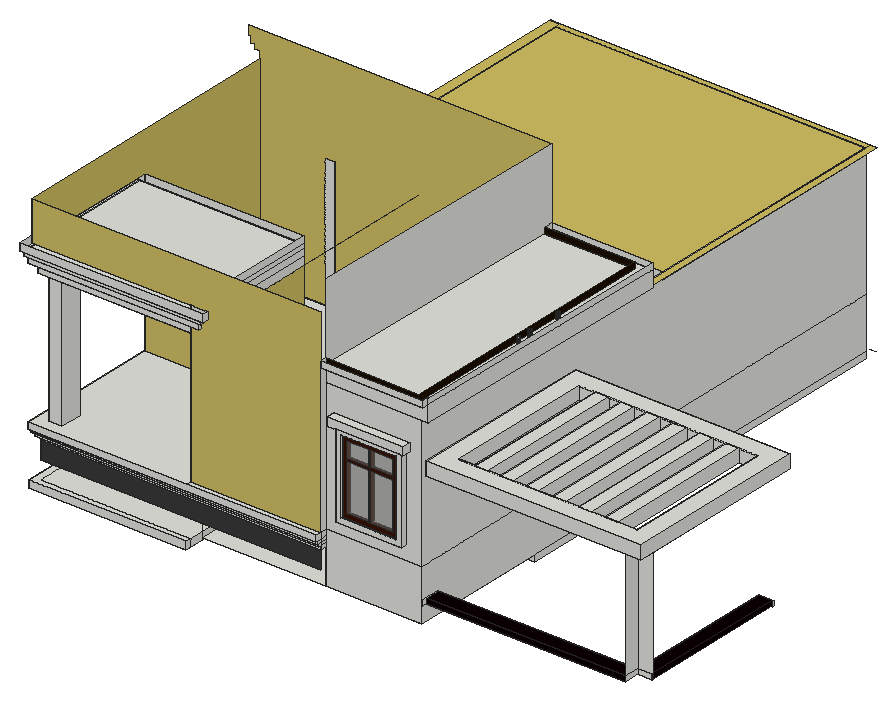
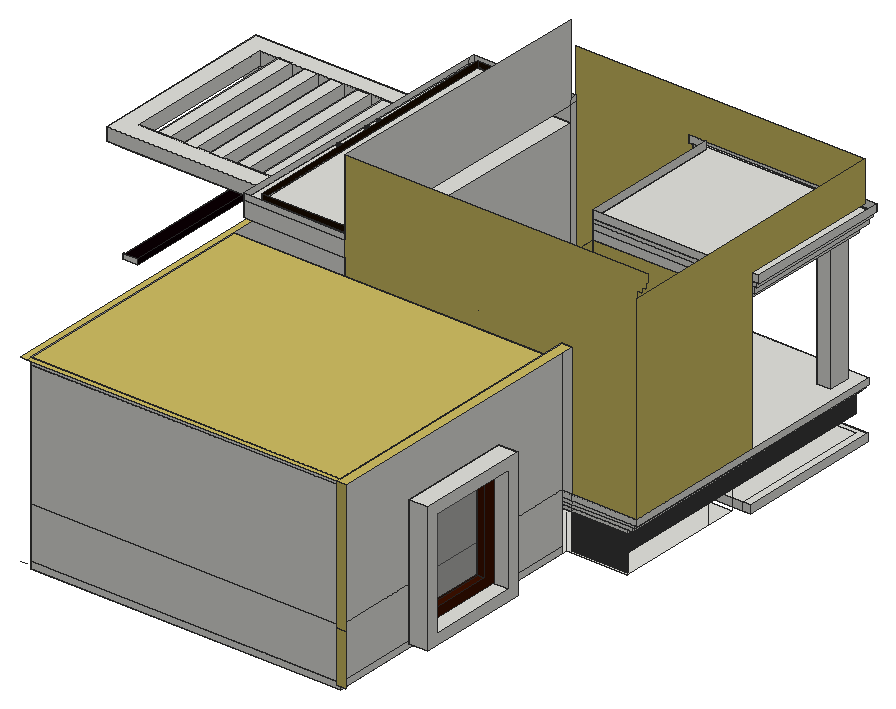
# SketchUp Ruby script. Lengths in inches.
U = 1.inch
M = Sketchup.active_model
def pt(a) = Geom::Point3d.new(a.map { |v| v * U })
def face(e, loops, mat)
  f = e.add_face(loops[0].map { |a| pt(a) })
  loops[1..].each { |l| e.add_face(l.map { |a| pt(a) }).erase! }
  f.material = f.back_material = mat if mat
  f
end
# faces: each face lists its corners as indices into pts; further lists are holes
def faces(e, pts, list, mat = nil) = list.each { |f| face(e, (f[0].is_a?(Array) ? f : [f]).map { |l| l.map { |i| pts[i] } }, mat) }
# xy, xz, yz: faces in a plane at the given z, y or x. An outline is a flat list of corners, or four numbers for a rectangle; further outlines are holes
def ring(l) = l.size == 4 ? [[l[0], l[1]], [l[2], l[1]], [l[2], l[3]], [l[0], l[3]]] : l.each_slice(2).to_a
def flat(e, list, mat, &to3) = list.each { |f| face(e, (f[0].is_a?(Array) ? f : [f]).map { |l| ring(l).map { |u, v| to3.(u, v) } }, mat) }
def xy(e, z, list, mat = nil) = flat(e, list, mat) { |x, y| [x, y, z] }
def xz(e, y, list, mat = nil) = flat(e, list, mat) { |x, z| [x, y, z] }
def yz(e, x, list, mat = nil) = flat(e, list, mat) { |y, z| [x, y, z] }
def lines(e, pts, list) = list.each { |a, b| e.add_line(pt(pts[a]), pt(pts[b])) }
# prism: a flat outline (further loops are holes) pulled along v
def prism(e, loops, v, mat = nil)
  f = face(e, loops, mat); d = Geom::Vector3d.new(v.map { |x| x * U })
  f.pushpull(f.normal.samedirection?(d) ? d.length : -d.length)
end
def box(e, o, s, mat = nil) = prism(e, [[o, [o[0] + s[0], o[1], o[2]], [o[0] + s[0], o[1] + s[1], o[2]], [o[0], o[1] + s[1], o[2]]]], [0, 0, s[2]], mat)
def at(x, y, z, deg = 0) = Geom::Transformation.translation(pt([x, y, z])) * Geom::Transformation.rotation(ORIGIN, Z_AXIS, deg.degrees)
def axes(o, x, y, z) = Geom::Transformation.new([*x, 0, *y, 0, *z, 0, *pt(o).to_a, 1])
def part(name) = M.definitions.add(name)
# library, detail: a bought-in or finely detailed component or shape, given as its bounding box
def library(name, o, s) = part(name).tap { |d| box(d.entities, o, s) }
def detail(e, o, s) = box(e.add_group.entities, o, s)
def put(e, d, t, mat = nil) = e.add_instance(d, t).tap { |i| i.material = mat if mat }
def group(e, t, mat = nil) = e.add_group.tap { |g| g.transformation = t; g.material = mat if mat }.entities
root = M.entities
M.materials.add("[Color C08]").color = [60, 17, 0]
M.materials.add("[Color D05]").color = [208, 191, 99]
M.materials.add("[Color E01]").color = [255, 255, 204]
M.materials.add("[Color M07]").color = [58, 58, 58]
M.materials.add("[Metal Seamed]").color = [11, 0, 4]
M.materials.add("[Metal Seamed]1").color = [28, 14, 0]
M.materials.add("[Translucent Glass Gray]").color = [128, 128, 128]
M.materials["[Translucent Glass Gray]"].alpha = 0.5
M.materials.add("[Wood Cherry Original]").color = [152, 86, 42]
c1 = part("Group\#2")
xy(c1.entities,0,[[0,0,43.625,4]],"[Color C08]")
xy(c1.entities,4.9,[[4.9,0,38.73,4]],"[Color C08]")
xy(c1.entities,53.48,[[4.9,0,38.73,4]],"[Color C08]")
xy(c1.entities,58.375,[[0,0,43.625,4]],"[Color C08]")
xz(c1.entities,0,[[[0,0,43.625,58.375],[4.9,4.9,38.73,53.48]]],"[Color C08]")
xz(c1.entities,0,[[4.9,4.9,38.73,53.48]],"[Translucent Glass Gray]")
xz(c1.entities,4,[[[0,0,43.625,58.375],[4.9,4.9,38.73,53.48]]],"[Color C08]")
yz(c1.entities,0,[[0,0,4,58.375]],"[Color C08]")
yz(c1.entities,4.9,[[0,4.9,4,53.48]],"[Color C08]")
yz(c1.entities,38.73,[[0,4.9,4,53.48]],"[Color C08]")
yz(c1.entities,43.625,[[0,0,4,58.375]],"[Color C08]")
c2 = part("Group\#1")
xy(c2.entities,0,[[0,0,6.3125,48]],"[Wood Cherry Original]")
xy(c2.entities,4.83,[[2.3125,4.83,3.9375,43.17]])
xy(c2.entities,4.83,[[0,4.83,2.3125,43.17],[3.9375,4.83,6.3125,43.17]],"[Wood Cherry Original]")
xy(c2.entities,79.17,[[2.3125,4.83,3.9375,43.17]])
xy(c2.entities,79.17,[[0,4.83,2.3125,43.17],[3.9375,4.83,6.3125,43.17]],"[Wood Cherry Original]")
xy(c2.entities,84,[[0,0,6.3125,48]],"[Wood Cherry Original]")
xz(c2.entities,0,[[0,0,6.3125,84]],"[Wood Cherry Original]")
xz(c2.entities,4.83,[[2.3125,4.83,3.9375,79.17]])
xz(c2.entities,4.83,[[0,4.83,2.3125,79.17],[3.9375,4.83,6.3125,79.17]],"[Wood Cherry Original]")
xz(c2.entities,43.17,[[2.3125,4.83,3.9375,79.17]])
xz(c2.entities,43.17,[[0,4.83,2.3125,79.17],[3.9375,4.83,6.3125,79.17]],"[Wood Cherry Original]")
xz(c2.entities,48,[[0,0,6.3125,84]],"[Wood Cherry Original]")
yz(c2.entities,0,[[[0,0,48,84],[4.83,4.83,43.17,79.17]]],"[Wood Cherry Original]")
yz(c2.entities,2.3125,[[7.68,9.76,40.37,11.76],[7.68,18.32,40.37,20.32],[7.68,27.01,40.37,29.01],[7.68,35.69,40.37,37.69],[7.68,44.38,40.37,46.38],
  [7.68,53.07,40.37,55.07],[7.68,61.76,40.37,63.76],[7.68,70.44,40.37,72.44]],"[Color E01]")
yz(c2.entities,2.3125,[[[4.83,4.83,43.17,79.17],[7.68,70.44,40.37,72.44],[7.68,61.76,40.37,63.76],[7.68,53.07,40.37,55.07],[7.68,44.38,40.37,46.38],[7.68,35.69,40.37,37.69],[7.68,27.01,40.37,29.01],[7.68,18.32,40.37,20.32],[7.68,9.76,40.37,11.76]]],"[Wood Cherry Original]")
yz(c2.entities,3.9375,[[4.83,4.83,43.17,79.17]],"[Wood Cherry Original]")
yz(c2.entities,6.3125,[[[0,0,48,84],[4.83,4.83,43.17,79.17]]],"[Wood Cherry Original]")
c3 = part("Group\#3")
xy(c3.entities,0,[[0,0,51.6875,4]],"[Color C08]")
xy(c3.entities,4.05,[[4.05,0,24.41,4],[24.41,0,26.55,4],[26.55,0,47.64,4]],"[Color C08]")
xy(c3.entities,49.59,[[4.05,0,24.41,4],[26.55,0,47.64,4]],"[Color C08]")
xy(c3.entities,51.6875,[[4.05,0,24.41,4],[26.55,0,47.64,4]],"[Color C08]")
xy(c3.entities,67.57,[[4.05,0,24.41,4],[26.55,0,47.64,4]],"[Color C08]")
xy(c3.entities,71.625,[[0,0,51.6875,4]],"[Color C08]")
xz(c3.entities,0,[[[0,0,51.6875,71.625],[4.05,4.05,4.05,49.59,24.41,49.59,24.41,4.05,26.55,4.05,26.55,49.59,47.64,49.59,47.64,4.05],[26.55,51.6875,47.64,67.57],[4.05,51.6875,24.41,67.57]]],"[Color C08]")
xz(c3.entities,0,[[4.05,4.05,24.41,49.59],[26.55,4.05,47.64,49.59],[4.05,51.6875,24.41,67.57],[26.55,51.6875,47.64,67.57]],"[Translucent Glass Gray]")
xz(c3.entities,4,[[[0,0,51.6875,71.625],[4.05,4.05,4.05,49.59,24.41,49.59,24.41,4.05,26.55,4.05,26.55,49.59,47.64,49.59,47.64,4.05],[26.55,51.6875,47.64,67.57],[4.05,51.6875,24.41,67.57]]],"[Color C08]")
yz(c3.entities,0,[[0,0,4,71.625]],"[Color C08]")
yz(c3.entities,4.05,[[0,4.05,4,49.59],[0,51.6875,4,67.57]],"[Color C08]")
yz(c3.entities,24.41,[[0,4.05,4,49.59],[0,51.6875,4,67.57]],"[Color C08]")
yz(c3.entities,26.55,[[0,4.05,4,49.59],[0,51.6875,4,67.57]],"[Color C08]")
yz(c3.entities,47.64,[[0,4.05,4,49.59],[0,51.6875,4,67.57]],"[Color C08]")
yz(c3.entities,51.6875,[[0,0,4,71.625]],"[Color C08]")
xy(root,425,[[14.875,61.97,14.875,195.41,17.375,195.41,17.375,63.91,21.75,63.91,21.75,61.97],[21.75,61.97,158,63.91],[17.375,63.91,158,195.41]])
xy(root,426,[[26.75,201.41,26.75,320.85,81.6875,320.85,81.6875,578.04,363.3125,578.04,363.3125,201.41]])
xy(root,432,[[14.875,61.97,158,61.97,158,67.28,21.75,67.28,21.75,195.41,14.875,195.41],[21.75,67.28,158,195.41],[164,73.28,164,201.41,277.42,201.41,275.92,73.28],[275.92,73.28,277.42,201.41,363.3125,201.41,363.3125,73.28],[277.42,201.41,363.3125,201.41,363.3125,578.04,81.6875,578.04,81.6875,326.53,278.88,326.53]])
xy(root,437.76,[[55.1875,409.72,72.6875,511.69]])
xy(root,447.65,[[55.1875,419.61,72.6875,501.8],[72.6875,419.61,81.6875,501.8]])
xy(root,450.5,[[505.19,75.15,505.97,75.25,506.69,75.55,507.3125,76.03,507.79,76.65,508.09,77.37,508.19,78.15,508.09,78.92,507.79,79.65,507.3125,80.27,506.69,80.75,505.97,81.05,505.19,81.15,504.42,81.05,503.69,80.75,503.07,80.27,502.59,79.65,502.29,78.92,502.19,78.15,502.29,77.37,502.59,76.65,503.07,76.03,503.69,75.55,504.42,75.25]])
xy(root,450.75,[[486.19,75.15,486.97,75.25,487.69,75.55,488.3125,76.03,488.79,76.65,489.09,77.37,489.19,78.15,489.09,78.92,488.79,79.65,488.3125,80.27,487.69,80.75,486.97,81.05,486.19,81.15,485.42,81.05,484.69,80.75,484.07,80.27,483.59,79.65,483.29,78.92,483.19,78.15,483.29,77.37,483.59,76.65,484.07,76.03,484.69,75.55,485.42,75.25]])
xy(root,451.5,[[554.92,112.25,555.73,112.35,556.48,112.66,557.13,113.16,557.625,113.81,557.9375,114.5625,558.04,115.37,557.9375,116.18,557.625,116.93,557.13,117.58,556.48,118.08,555.73,118.39,554.92,118.5,554.11,118.39,553.36,118.08,552.71,117.58,552.21,116.93,551.9,116.18,551.79,115.37,551.9,114.5625,552.21,113.81,552.71,113.16,553.36,112.66,554.11,112.35],[554.92,166.43,555.73,166.54,556.48,166.85,557.13,167.35,557.625,168,557.9375,168.75,558.04,169.56,557.9375,170.37,557.625,171.12,557.13,171.77,556.48,172.26,555.73,172.58,554.92,172.68,554.11,172.58,553.36,172.26,552.71,171.77,552.21,171.12,551.9,170.37,551.79,169.56,551.9,168.75,552.21,168,552.71,167.35,553.36,166.85,554.11,166.54]])
xy(root,451.5625,[[[369.3125,70.97,550.8125,84.66],[383.69,75.15,384.47,75.25,385.19,75.55,385.8125,76.03,386.29,76.65,386.59,77.37,386.69,78.15,386.59,78.92,386.29,79.65,385.8125,80.27,385.19,80.75,384.47,81.05,383.69,81.15,382.92,81.05,382.19,80.75,381.57,80.27,381.09,79.65,380.79,78.92,380.69,78.15,380.79,77.37,381.09,76.65,381.57,76.03,382.19,75.55,382.92,75.25],[404.19,75.15,404.97,75.25,405.69,75.55,406.3125,76.03,406.79,76.65,407.09,77.37,407.19,78.15,407.09,78.92,406.79,79.65,406.3125,80.27,405.69,80.75,404.97,81.05,404.19,81.15,403.42,81.05,402.69,80.75,402.07,80.27,401.59,79.65,401.29,78.92,401.19,78.15,401.29,77.37,401.59,76.65,402.07,76.03,402.69,75.55,403.42,75.25],[445.19,75.15,445.97,75.25,446.69,75.55,447.3125,76.03,447.79,76.65,448.09,77.37,448.19,78.15,448.09,78.92,447.79,79.65,447.3125,80.27,446.69,80.75,445.97,81.05,445.19,81.15,444.42,81.05,443.69,80.75,443.07,80.27,442.59,79.65,442.29,78.92,442.19,78.15,442.29,77.37,442.59,76.65,443.07,76.03,443.69,75.55,444.42,75.25]],[550.8125,84.66,550.8125,222.34,564.5,222.34,564.5,221.65,563.5625,221.65,563.5625,84.66],[554.92,94.18,555.73,94.29,556.48,94.6,557.13,95.1,557.625,95.75,557.9375,96.5,558.04,97.31,557.9375,98.12,557.625,98.87,557.13,99.52,556.48,100.01,555.73,100.33,554.92,100.43,554.11,100.33,553.36,100.01,552.71,99.52,552.21,98.87,551.9,98.12,551.79,97.31,551.9,96.5,552.21,95.75,552.71,95.1,553.36,94.6,554.11,94.29]])
xy(root,451.6875,[[465.69,75.15,466.47,75.25,467.19,75.55,467.8125,76.03,468.29,76.65,468.59,77.37,468.69,78.15,468.59,78.92,468.29,79.65,467.8125,80.27,467.19,80.75,466.47,81.05,465.69,81.15,464.92,81.05,464.19,80.75,463.57,80.27,463.09,79.65,462.79,78.92,462.69,78.15,462.79,77.37,463.09,76.65,463.57,76.03,464.19,75.55,464.92,75.25]])
xy(root,451.75,[[554.92,148.37,555.73,148.48,556.48,148.79,557.13,149.29,557.625,149.93,557.9375,150.6875,558.04,151.5,557.9375,152.3,557.625,153.06,557.13,153.71,556.48,154.2,555.73,154.51,554.92,154.62,554.11,154.51,553.36,154.2,552.71,153.71,552.21,153.06,551.9,152.3,551.79,151.5,551.9,150.6875,552.21,149.93,552.71,149.29,553.36,148.79,554.11,148.48]])
xy(root,452.1875,[[527.82,75.15,528.59,75.25,529.32,75.55,529.9375,76.03,530.42,76.65,530.72,77.37,530.82,78.15,530.72,78.92,530.42,79.65,529.9375,80.27,529.32,80.75,528.59,81.05,527.82,81.15,527.04,81.05,526.32,80.75,525.7,80.27,525.22,79.65,524.92,78.92,524.82,78.15,524.92,77.37,525.22,76.65,525.7,76.03,526.32,75.55,527.04,75.25]])
xy(root,452.4375,[[554.92,201.87,555.73,201.98,556.48,202.29,557.13,202.79,557.625,203.43,557.9375,204.1875,558.04,205,557.9375,205.8,557.625,206.56,557.13,207.21,556.48,207.7,555.73,208.01,554.92,208.12,554.11,208.01,553.36,207.7,552.71,207.21,552.21,206.56,551.9,205.8,551.79,205,551.9,204.1875,552.21,203.43,552.71,202.79,553.36,202.29,554.11,201.98]])
xy(root,452.5,[[554.92,184.5,555.73,184.6,556.48,184.91,557.13,185.41,557.625,186.06,557.9375,186.8125,558.04,187.62,557.9375,188.43,557.625,189.18,557.13,189.83,556.48,190.33,555.73,190.64,554.92,190.75,554.11,190.64,553.36,190.33,552.71,189.83,552.21,189.18,551.9,188.43,551.79,187.62,551.9,186.8125,552.21,186.06,552.71,185.41,553.36,184.91,554.11,184.6]])
xy(root,453.1875,[[554.92,130.31,555.73,130.41,556.48,130.73,557.13,131.22,557.625,131.87,557.9375,132.625,558.04,133.43,557.9375,134.24,557.625,135,557.13,135.64,556.48,136.14,555.73,136.45,554.92,136.56,554.11,136.45,553.36,136.14,552.71,135.64,552.21,135,551.9,134.24,551.79,133.43,551.9,132.625,552.21,131.87,552.71,131.22,553.36,130.73,554.11,130.41]])
xy(root,454.875,[[424.69,75.15,425.47,75.25,426.19,75.55,426.8125,76.03,427.29,76.65,427.59,77.37,427.69,78.15,427.59,78.92,427.29,79.65,426.8125,80.27,426.19,80.75,425.47,81.05,424.69,81.15,423.92,81.05,423.19,80.75,422.57,80.27,422.09,79.65,421.79,78.92,421.69,78.15,421.79,77.37,422.09,76.65,422.57,76.03,423.19,75.55,423.92,75.25]])
xy(root,456,[[369.3125,70.97,550.8125,84.66],[550.8125,84.66,563.5625,84.66,563.5625,221.65,564.5,221.65,564.5,222.34,550.8125,222.34]],"[Metal Seamed]")
xy(root,464.125,[[21.75,67.22,158,67.28],[158,67.22,275.92,67.28],[21.75,67.28,21.75,326.53,278.88,326.53,277.42,201.41,275.92,73.28,275.92,67.28]])
xy(root,467.3125,[[17.25,65.35,21.75,326.53],[21.75,65.35,275.92,67.22],[21.75,67.22,21.75,326.53,278.88,326.53,275.92,73.28,275.92,67.22]])
xy(root,469.8125,[[15,64.03,15,326.53,17.25,326.53,17.25,65.35,21.75,65.35,21.75,64.03],[21.75,64.03,275.92,65.35],[17.25,65.35,17.25,326.53,278.88,326.53,275.92,73.28,275.92,65.35]])
xy(root,472.625,[[13.375,62.47,13.375,326.53,15,326.53,15,64.03,21.75,64.03,21.75,62.47],[21.75,62.47,275.92,64.03]])
xy(root,478.25,[[[13.375,62.47,158,62.47,158,120.11,178.625,120.11,178.625,168.11,158,168.11,158,195.41,13.375,195.41],[24.07,73.08,36.38,92.83]],[158,62.47,275.92,67.28],[158,67.28,158,120.11,178.625,120.11,178.625,168.11,158,168.11,158,326.53,278.88,326.53,275.92,73.28,275.92,67.28],[24.07,73.08,36.38,92.83],[13.375,195.41,158,326.53]])
xy(root,495.55,[[294.14,62.22,353.83,67.28]])
xy(root,500.37,[[298.95,62.22,349.02,67.28]])
xy(root,545.15,[[55.1875,419.61,72.6875,501.8],[72.6875,419.61,81.6875,501.8]])
xy(root,555.04,[[55.1875,409.72,72.6875,511.69]])
xy(root,555.625,[[369.3125,70.97,369.3125,240.85,545.3,240.85,545.3,224.6,385.56,224.6,385.56,87.22,519.19,87.22,519.19,87.1,531.19,87.1,531.19,87.22,548.25,87.22,548.25,221.65,564.5,221.65,564.5,84.66,550.8125,84.66,550.8125,70.97],[550.8125,70.97,564.5,84.66],[519.19,87.1,531.19,87.22],[400.38,87.22,412.38,224.6],[423.69,87.22,435.69,224.6],
  [447.13,87.22,459.13,224.6],[471.32,87.22,483.32,224.6],[495.07,87.22,507.07,224.6],[519.19,87.22,531.19,224.6],[545.3,221.65,548.25,224.6],
  [548.25,221.65,548.25,224.6,545.3,224.6,545.3,240.85,564.5,240.85,564.5,221.65]])
xy(root,562.25,[[158,120.11,178.625,168.11]])
xy(root,567.625,[[[369.3125,70.97,564.5,240.85],[385.56,87.22,548.25,224.6]],[519.19,87.1,531.19,87.22],[400.38,87.22,412.38,224.6],[423.69,87.22,435.69,224.6],[447.13,87.22,459.13,224.6],
  [471.32,87.22,483.32,224.6],[495.07,87.22,507.07,224.6],[519.19,87.22,531.19,224.6]])
xy(root,568.31,[[298.95,62.22,349.02,67.28]])
xy(root,572.84,[[287.75,59.28,294.14,67.28],[353.83,59.28,357.625,67.28]])
xy(root,573.125,[[294.14,59.28,353.83,62.22],[294.14,62.22,353.83,67.28]])
xy(root,580.15,[[287.75,59.28,357.625,67.28]])
xy(root,592.25,[[81.6875,347.04,363.3125,578.04]])
xy(root,598.25,[[[16.875,69.28,158,195.41],[24.07,73.08,36.38,92.83]],[369.3125,72.19,369.3125,325.48,363.3125,325.55,363.3125,73.28,275.92,73.28],[369.3125,72.19,369.3125,325.48,372.33,325.44,369.37,72.19],[275.92,73.28,278.88,326.53,363.3125,325.55,363.3125,73.28]])
xy(root,598.25,[[369.3125,325.48,369.3125,582.91,363.3125,582.91,363.3125,325.55],[72.6875,326.53,81.6875,582.91],[81.6875,347.04,363.3125,578.04],[81.6875,578.04,363.3125,582.91]],"[Color D05]")
xy(root,605.9375,[[10.9375,65.41,10.9375,195.41,16.875,195.41,16.875,69.28,13.375,69.28,13.375,65.41],[13.375,65.41,13.375,69.28,158,69.28,158,67.28,167.0625,67.28,167.0625,65.41],[16.875,69.28,158,195.41]])
xy(root,611.625,[[8.8125,63.78,8.8125,195.41,10.9375,195.41,10.9375,65.41,13.375,65.41,13.375,63.78],[13.375,63.78,169.8125,65.41],[10.9375,65.41,10.9375,195.41,158,195.41,158,67.28,167.0625,67.28,167.0625,65.41],[167.0625,65.41,169.8125,67.28]])
xy(root,612.6875,[[361.23,72.29,361.23,318.35,278.78,318.35,275.92,73.28],[363.55,181.41,363.21,181.5,362.92,181.67,362.67,181.91,362.5,182.21,362.41,182.54,362.41,182.88,362.5,183.21,362.67,183.51,362.91,183.75,363.2,183.92,363.54,184.01,363.88,184.01,364.21,183.93,364.51,183.76,364.75,183.51,364.92,183.22,365.01,182.89,365.01,182.55,364.93,182.21,364.76,181.92,364.51,181.67,364.22,181.5,363.89,181.41],[363.55,194.29,363.21,194.37,362.92,194.54,362.67,194.78,362.5,195.08,362.41,195.41,362.41,195.75,362.5,196.08,362.67,196.38,362.91,196.625,363.2,196.8,363.54,196.89,363.88,196.89,364.21,196.8,364.51,196.63,364.75,196.39,364.92,196.09,365.01,195.76,365.01,195.42,364.93,195.09,364.76,194.79,364.51,194.55,364.22,194.375,363.89,194.29],[363.55,226.47,363.21,226.56,362.92,226.73,362.67,226.97,362.5,227.27,362.41,227.6,362.41,227.94,362.5,228.27,362.67,228.57,362.91,228.8125,363.2,228.99,363.54,229.08,363.88,229.08,364.21,228.99,364.51,228.82,364.75,228.58,364.92,228.28,365.01,227.95,365.01,227.61,364.93,227.28,364.76,226.98,364.51,226.74,364.22,226.5625,363.89,226.47]])
xy(root,612.8125,[[275.92,67.28,275.92,73.28,361.23,72.29,369.3125,72.19,369.3125,67.28],[369.3125,72.19,361.23,72.29,361.23,318.35,278.78,318.35,278.88,326.53,372.33,325.44,369.37,72.19]])
xy(root,615.5,[[6.875,62.22,6.875,195.41,8.8125,195.41,8.8125,63.78,13.375,63.78,13.375,62.22],[13.375,62.22,173.1875,63.78],[8.8125,63.78,8.8125,195.41,158,195.41,158,67.28,169.8125,67.28,169.8125,63.78],[169.8125,63.78,173.1875,67.28]])
xz(root,59.28,[[287.75,572.84,294.14,572.84,294.14,573.125,353.83,573.125,353.83,572.84,357.625,572.84,357.625,580.15,287.75,580.15]])
xz(root,61.97,[[14.875,425,158,432]])
xz(root,62.22,[[[294.14,495.55,353.83,573.125],[298.95,500.37,349.02,568.31]],[6.875,615.5,173.1875,622.25]])
xz(root,62.47,[[13.375,472.625,275.92,478.25]])
xz(root,63.78,[[8.8125,611.625,169.8125,615.5]])
xz(root,64.03,[[15,469.8125,275.92,472.625]])
xz(root,65.35,[[17.25,467.3125,275.92,469.8125]])
xz(root,65.41,[[10.9375,605.9375,167.0625,611.625]])
xz(root,67.22,[[21.75,464.125,275.92,467.3125]])
xz(root,67.28,[[[294.14,495.55,353.83,572.84],[298.95,500.37,349.02,568.31]],[298.95,500.37,349.02,568.31],[294.14,572.84,353.83,573.125],[158,605.9375,167.0625,611.625],[158,611.625,169.8125,615.5],
  [275.92,612.8125,369.3125,618.25],[158,615.5,173.1875,622.25]])
xz(root,67.28,[[158,478.25,275.92,478.25,275.92,658.25,13.375,658.25,13.375,622.25,173.1875,622.25,173.1875,615.5,169.8125,615.5,169.8125,611.625,167.0625,611.625,167.0625,605.9375,158,605.9375]],"[Color D05]")
xz(root,67.28,[[21.75,448.0625,275.92,464.125]],"[Color M07]")
xz(root,69.28,[[16.875,598.25,158,605.9375]])
xz(root,70.97,[[369.3125,555.625,564.5,567.625]])
xz(root,70.97,[[369.3125,451.5625,550.8125,456]],"[Metal Seamed]")
xz(root,72.19,[[369.3125,598.25,369.37,612.8125],[369.3125,612.8125,369.37,618.25]])
xz(root,73.08,[[24.07,478.25,36.38,598.25]])
xz(root,73.28,[[275.92,432,363.3125,478.25],[275.92,478.25,363.3125,598.25]])
xz(root,84.66,[[550.8125,451.5625,563.5625,456],[563.5625,451.5625,564.5,456],[550.8125,456,564.5,555.625]])
xz(root,84.66,[[369.3125,451.5625,550.8125,456]],"[Metal Seamed]")
xz(root,87.1,[[519.19,555.625,531.19,567.625]])
xz(root,87.22,[[385.56,555.625,400.38,567.625],[400.38,555.625,412.38,567.625],[412.38,555.625,423.69,567.625],[423.69,555.625,435.69,567.625],[435.69,555.625,447.13,567.625],
  [447.13,555.625,459.13,567.625],[459.13,555.625,471.32,567.625],[471.32,555.625,483.32,567.625],[483.32,555.625,495.07,567.625],[495.07,555.625,507.07,567.625],
  [507.07,555.625,548.25,567.625]])
xz(root,92.83,[[24.07,478.25,36.38,598.25]])
xz(root,120.11,[[158,478.25,178.625,562.25]])
xz(root,168.11,[[158,478.25,178.625,562.25]])
xz(root,181.41,[[363.55,612.6875,363.89,618.25]])
xz(root,184.01,[[363.54,612.6875,363.88,618.25]])
xz(root,194.29,[[363.55,612.6875,363.89,618.25]])
xz(root,195.41,[[14.875,425,21.75,432],[21.75,425,158,432],[13.375,598.25,16.875,605.9375],[16.875,598.25,158,605.9375],[10.9375,605.9375,13.375,611.625],
  [13.375,605.9375,158,611.625],[8.8125,611.625,13.375,615.5],[13.375,611.625,158,615.5],[6.875,615.5,13.375,622.25],[13.375,615.5,158,622.25]])
xz(root,195.41,[[13.375,478.25,158,598.25]],"[Color D05]")
xz(root,196.89,[[363.54,612.6875,363.88,618.25]])
xz(root,201.41,[[164,426,363.3125,432]])
xz(root,221.65,[[563.5625,451.5625,564.5,456]])
xz(root,222.34,[[550.8125,451.5625,564.5,456]])
xz(root,224.6,[[385.56,555.625,400.38,567.625],[400.38,555.625,412.38,567.625],[412.38,555.625,423.69,567.625],[423.69,555.625,435.69,567.625],[435.69,555.625,447.13,567.625],
  [447.13,555.625,459.13,567.625],[459.13,555.625,471.32,567.625],[471.32,555.625,483.32,567.625],[483.32,555.625,495.07,567.625],[495.07,555.625,507.07,567.625],
  [507.07,555.625,519.19,567.625],[519.19,555.625,531.19,567.625],[531.19,555.625,548.25,567.625]])
xz(root,226.47,[[363.55,612.6875,363.89,618.25]])
xz(root,229.08,[[363.54,612.6875,363.88,618.25]])
xz(root,240.85,[[369.3125,555.625,564.5,567.625]])
xz(root,318.35,[[278.78,612.6875,361.23,612.8125]])
xz(root,318.35,[[278.78,612.8125,361.23,618.25]],"[Metal Seamed]1")
xz(root,326.53,[[81.6875,432,278.88,464.125],[21.75,464.125,72.6875,467.3125],[72.6875,464.125,81.6875,467.3125],[81.6875,464.125,278.88,467.3125],[17.25,467.3125,72.6875,469.8125],
  [72.6875,467.3125,81.6875,469.8125],[81.6875,467.3125,278.88,469.8125],[15,469.8125,72.6875,472.625],[72.6875,469.8125,81.6875,472.625],[81.6875,469.8125,278.88,472.625],
  [13.375,472.625,72.6875,478.25],[72.6875,472.625,81.6875,478.25],[81.6875,472.625,278.88,478.25],[72.6875,478.25,81.6875,598.25]])
xz(root,326.53,[[13.375,478.25,13.375,665,8.6875,665,8.6875,669.0625,5.625,669.0625,5.625,674.375,3.625,674.375,3.625,682.25,278.88,682.25,278.88,478.25,81.6875,478.25,81.6875,598.25,72.6875,598.25,72.6875,478.25]],"[Color D05]")
xz(root,326.53,[[21.75,432,72.6875,464.125]],"[Color M07]")
xz(root,347.04,[[81.6875,592.25,363.3125,598.25]])
xz(root,409.72,[[55.1875,437.76,72.6875,555.04]])
xz(root,419.61,[[55.1875,447.65,72.6875,545.15],[72.6875,447.65,81.6875,545.15]])
xz(root,501.8,[[55.1875,447.65,72.6875,545.15],[72.6875,447.65,81.6875,545.15]])
xz(root,511.69,[[55.1875,437.76,72.6875,555.04]])
xz(root,578.04,[[81.6875,426,363.3125,432],[81.6875,432,363.3125,478.25],[81.6875,478.25,363.3125,592.25],[81.6875,592.25,363.3125,598.25]])
xz(root,582.91,[[72.6875,432,81.6875,478.25],[72.6875,478.25,81.6875,598.25]],"[Color D05]")
yz(root,6.875,[[62.22,615.5,195.41,622.25]])
yz(root,8.8125,[[63.78,611.625,195.41,615.5]])
yz(root,10.9375,[[65.41,605.9375,195.41,611.625]])
yz(root,13.375,[[62.47,472.625,326.53,478.25]])
yz(root,13.375,[[195.41,478.25,195.41,622.25,67.28,622.25,67.28,658.25,326.53,658.25,326.53,478.25]],"[Color D05]")
yz(root,14.875,[[61.97,425,195.41,432]])
yz(root,15,[[64.03,469.8125,326.53,472.625]])
yz(root,16.875,[[69.28,598.25,195.41,605.9375]])
yz(root,17.25,[[65.35,467.3125,326.53,469.8125]])
yz(root,21.75,[[67.22,464.125,326.53,467.3125]])
yz(root,21.75,[[67.28,448.0625,326.53,464.125]],"[Color M07]")
yz(root,24.07,[[73.08,478.25,92.83,598.25]])
yz(root,36.38,[[73.08,478.25,92.83,598.25]])
yz(root,55.1875,[[[409.72,437.76,511.69,555.04],[419.61,447.65,501.8,545.15]]])
yz(root,72.6875,[[[409.72,437.76,511.69,555.04],[419.61,447.65,501.8,545.15]]])
yz(root,81.6875,[[326.53,426,578.04,432],[326.53,432,578.04,432,578.04,478.25,501.8,478.25,501.8,447.65,419.61,447.65,419.61,478.25,326.53,478.25],[419.61,447.65,501.8,478.25],[326.53,478.25,419.61,478.25,419.61,545.15,501.8,545.15,501.8,478.25,578.04,478.25,578.04,592.25,347.04,592.25,347.04,598.25,326.53,598.25],[419.61,478.25,501.8,545.15],
  [347.04,592.25,578.04,598.25]])
yz(root,158,[[61.97,425,67.28,432],[67.28,425,195.41,432],[69.28,598.25,195.41,605.9375],[67.28,605.9375,195.41,611.625],[67.28,611.625,195.41,615.5],
  [67.28,615.5,195.41,622.25]])
yz(root,158,[[67.28,478.25,67.28,605.9375,69.28,605.9375,69.28,598.25,195.41,598.25,195.41,478.25,168.11,478.25,168.11,562.25,120.11,562.25,120.11,478.25]],"[Color D05]")
yz(root,167.0625,[[65.41,605.9375,67.28,611.625]])
yz(root,169.8125,[[63.78,611.625,67.28,615.5]])
yz(root,173.1875,[[62.22,615.5,67.28,622.25]])
yz(root,178.625,[[120.11,478.25,168.11,562.25]])
yz(root,275.92,[[67.22,464.125,67.28,467.3125],[67.28,464.125,73.28,467.3125],[65.35,467.3125,67.28,469.8125],[67.28,467.3125,73.28,469.8125],[64.03,469.8125,67.28,472.625],
  [67.28,469.8125,73.28,472.625],[62.47,472.625,67.28,478.25],[67.28,472.625,73.28,478.25],[67.28,478.25,73.28,612.8125],[67.28,612.8125,73.28,618.25]])
yz(root,287.75,[[59.28,572.84,67.28,580.15]])
yz(root,294.14,[[62.22,495.55,67.28,572.84],[59.28,572.84,62.22,573.125],[62.22,572.84,67.28,573.125]])
yz(root,298.95,[[62.22,500.37,67.28,568.31]])
yz(root,349.02,[[62.22,500.37,67.28,568.31]])
yz(root,353.83,[[62.22,495.55,67.28,572.84],[59.28,572.84,62.22,573.125],[62.22,572.84,67.28,573.125]])
yz(root,357.625,[[59.28,572.84,67.28,580.15]])
yz(root,361.23,[[72.29,612.6875,318.35,612.8125]])
yz(root,361.23,[[72.29,612.8125,318.35,618.25]],"[Metal Seamed]1")
yz(root,362.41,[[182.54,612.6875,182.88,618.25],[195.41,612.6875,195.75,618.25],[227.6,612.6875,227.94,618.25]])
yz(root,363.3125,[[201.41,426,578.04,432],[73.28,432,578.04,478.25],[73.28,478.25,73.28,598.25,347.04,598.25,347.04,592.25,578.04,592.25,578.04,478.25],[347.04,592.25,578.04,598.25]])
yz(root,365.01,[[182.55,612.6875,182.89,618.25],[195.42,612.6875,195.76,618.25],[227.61,612.6875,227.95,618.25]])
yz(root,369.3125,[[67.28,451.5625,70.97,456],[70.97,451.5625,84.66,456],[70.97,555.625,113.66,567.625],[113.66,555.625,119.66,567.625],[119.66,555.625,195.41,567.625],
  [195.41,555.625,240.85,567.625],[67.28,612.8125,72.19,618.25]])
yz(root,385.56,[[87.22,555.625,224.6,567.625]])
yz(root,400.38,[[87.22,555.625,224.6,567.625]])
yz(root,412.38,[[87.22,555.625,224.6,567.625]])
yz(root,423.69,[[87.22,555.625,224.6,567.625]])
yz(root,435.69,[[87.22,555.625,224.6,567.625]])
yz(root,447.13,[[87.22,555.625,224.6,567.625]])
yz(root,459.13,[[87.22,555.625,224.6,567.625]])
yz(root,471.32,[[87.22,555.625,224.6,567.625]])
yz(root,483.32,[[87.22,555.625,224.6,567.625]])
yz(root,495.07,[[87.22,555.625,224.6,567.625]])
yz(root,507.07,[[87.22,555.625,224.6,567.625]])
yz(root,519.19,[[87.1,555.625,224.6,567.625]])
yz(root,531.19,[[87.1,555.625,224.6,567.625]])
yz(root,548.25,[[87.22,555.625,224.6,567.625]])
yz(root,550.8125,[[70.97,451.5625,84.66,456],[70.97,456,84.66,555.625]])
yz(root,550.8125,[[84.66,451.5625,222.34,456]],"[Metal Seamed]")
yz(root,563.5625,[[84.66,451.5625,221.65,456]],"[Metal Seamed]")
yz(root,564.5,[[221.65,451.5625,222.34,456],[70.97,555.625,240.85,567.625]])
p = [[275.92,73.28,432],[277.42,201.41,432],[277.42,201.41,464.125],[275.92,73.28,464.125],[278.88,326.53,432],[278.88,326.53,464.125],
  [278.88,326.53,467.3125],[275.92,73.28,467.3125],[278.88,326.53,469.8125],[275.92,73.28,469.8125],[275.92,73.28,472.625],[278.88,326.53,472.625],
  [278.88,326.53,478.25],[275.92,73.28,478.25],[278.88,326.53,598.25],[275.92,73.28,598.25],[369.3125,72.19,598.25],[369.3125,72.19,612.8125],
  [361.23,72.29,612.8125],[361.23,72.29,612.6875],[275.92,73.28,612.6875],[369.37,72.19,598.25],[372.33,325.44,598.25],[372.33,325.44,612.8125],
  [369.37,72.19,612.8125],[278.88,326.53,612.8125],[369.3125,325.48,598.25],[363.3125,325.55,598.25],[275.92,73.28,612.8125],[278.88,326.53,618.25],
  [278.88,326.53,682.25],[275.92,73.28,682.25],[275.92,73.28,678.3125],[275.92,73.28,674.375],[275.92,73.28,670.37],[275.92,73.28,666.66],
  [275.92,73.28,618.25],[278.78,318.35,612.6875],[278.78,318.35,612.8125],[278.78,318.35,618.25],[278.79,318.92,618.25],[278.8125,320.82,618.25],
  [363.55,181.41,618.25],[363.21,181.5,618.25],[363.21,181.5,612.6875],[363.55,181.41,612.6875],[364.22,181.5,618.25],[363.89,181.41,618.25],
  [363.89,181.41,612.6875],[364.22,181.5,612.6875],[362.92,181.67,618.25],[362.92,181.67,612.6875],[364.51,181.67,618.25],[364.51,181.67,612.6875],
  [362.67,181.91,618.25],[362.67,181.91,612.6875],[364.76,181.92,618.25],[364.76,181.92,612.6875],[362.5,182.21,618.25],[362.5,182.21,612.6875],
  [364.93,182.21,618.25],[364.93,182.21,612.6875],[362.41,182.54,618.25],[362.41,182.54,612.6875],[365.01,182.55,618.25],[365.01,182.55,612.6875],
  [362.41,182.88,618.25],[362.5,183.21,618.25],[362.5,183.21,612.6875],[362.41,182.88,612.6875],[364.92,183.22,618.25],[365.01,182.89,618.25],
  [365.01,182.89,612.6875],[364.92,183.22,612.6875],[362.67,183.51,618.25],[362.67,183.51,612.6875],[364.75,183.51,618.25],[364.75,183.51,612.6875],
  [362.91,183.75,618.25],[362.91,183.75,612.6875],[364.51,183.76,618.25],[364.51,183.76,612.6875],[363.2,183.92,618.25],[363.2,183.92,612.6875],
  [364.21,183.93,618.25],[364.21,183.93,612.6875],[363.54,184.01,618.25],[363.54,184.01,612.6875],[363.88,184.01,618.25],[363.88,184.01,612.6875],
  [363.55,194.29,618.25],[363.21,194.37,618.25],[363.21,194.37,612.6875],[363.55,194.29,612.6875],[364.22,194.375,618.25],[363.89,194.29,618.25],
  [363.89,194.29,612.6875],[364.22,194.375,612.6875],[362.92,194.54,618.25],[362.92,194.54,612.6875],[364.51,194.55,618.25],[364.51,194.55,612.6875],
  [362.67,194.78,618.25],[362.67,194.78,612.6875],[364.76,194.79,618.25],[364.76,194.79,612.6875],[362.5,195.08,618.25],[362.5,195.08,612.6875],
  [364.93,195.09,618.25],[364.93,195.09,612.6875],[362.41,195.41,618.25],[362.41,195.41,612.6875],[365.01,195.42,618.25],[365.01,195.42,612.6875],
  [362.41,195.75,618.25],[362.5,196.08,618.25],[362.5,196.08,612.6875],[362.41,195.75,612.6875],[364.92,196.09,618.25],[365.01,195.76,618.25],
  [365.01,195.76,612.6875],[364.92,196.09,612.6875],[362.67,196.38,618.25],[362.67,196.38,612.6875],[364.75,196.39,618.25],[364.75,196.39,612.6875],
  [362.91,196.625,618.25],[362.91,196.625,612.6875],[364.51,196.63,618.25],[364.51,196.63,612.6875],[363.2,196.8,618.25],[363.2,196.8,612.6875],
  [364.21,196.8,618.25],[364.21,196.8,612.6875],[363.54,196.89,618.25],[363.54,196.89,612.6875],[363.88,196.89,618.25],[363.88,196.89,612.6875],
  [363.55,226.47,618.25],[363.21,226.56,618.25],[363.21,226.56,612.6875],[363.55,226.47,612.6875],[364.22,226.5625,618.25],[363.89,226.47,618.25],
  [363.89,226.47,612.6875],[364.22,226.5625,612.6875],[362.92,226.73,618.25],[362.92,226.73,612.6875],[364.51,226.74,618.25],[364.51,226.74,612.6875],
  [362.67,226.97,618.25],[362.67,226.97,612.6875],[364.76,226.98,618.25],[364.76,226.98,612.6875],[362.5,227.27,618.25],[362.5,227.27,612.6875],
  [364.93,227.28,618.25],[364.93,227.28,612.6875],[362.41,227.6,618.25],[362.41,227.6,612.6875],[365.01,227.61,618.25],[365.01,227.61,612.6875],
  [362.41,227.94,618.25],[362.5,228.27,618.25],[362.5,228.27,612.6875],[362.41,227.94,612.6875],[364.92,228.28,618.25],[365.01,227.95,618.25],
  [365.01,227.95,612.6875],[364.92,228.28,612.6875],[362.67,228.57,618.25],[362.67,228.57,612.6875],[364.75,228.58,618.25],[364.75,228.58,612.6875],
  [362.91,228.8125,618.25],[362.91,228.8125,612.6875],[364.51,228.82,618.25],[364.51,228.82,612.6875],[363.2,228.99,618.25],[363.2,228.99,612.6875],
  [364.21,228.99,618.25],[364.21,228.99,612.6875],[363.54,229.08,618.25],[363.54,229.08,612.6875],[363.88,229.08,618.25],[363.88,229.08,612.6875],
  [372.33,325.44,618.25],[369.37,72.19,618.25],[361.23,72.29,618.25],[158,195.41,432],[164,195.41,432],[363.3125,582.91,432],
  [369.3125,582.91,432],[26.75,320.85,426],[26.75,320.85,457.6875],[81.6875,320.85,426],[81.6875,320.85,457.6875],[26.75,228.85,457.6875],
  [26.75,228.85,426],[26.75,201.41,426],[26.75,201.41,457.6875],[164,73.28,432],[164,73.28,457.6875],[21.75,195.41,467.3125],
  [21.75,195.41,478.25],[158,195.41,598.25],[158,326.53,598.25]]
faces(root,p,[[0,1,2,3],[1,4,5,2],[5,6,7,3,2],[6,8,9,7],[10,9,8,11],[12,13,10,11],[13,12,14,15],[15,16,17,18,19,20],
  [21,22,23,24],[14,25,23,22,26,27],[18,28,20,19],[29,30,31,32,33,34,35,36,28,20,37,38,39,40,41],[42,43,44,45],[46,47,48,49],[43,50,51,44],[52,46,49,53],
  [50,54,55,51],[56,52,53,57],[54,58,59,55],[60,56,57,61],[58,62,63,59],[64,60,61,65],[66,67,68,69],[70,71,72,73],
  [67,74,75,68],[76,70,73,77],[74,78,79,75],[80,76,77,81],[78,82,83,79],[84,80,81,85],[82,86,87,83],[88,84,85,89],
  [90,91,92,93],[94,95,96,97],[91,98,99,92],[100,94,97,101],[98,102,103,99],[104,100,101,105],[102,106,107,103],[108,104,105,109],
  [106,110,111,107],[112,108,109,113],[114,115,116,117],[118,119,120,121],[115,122,123,116],[124,118,121,125],[122,126,127,123],[128,124,125,129],
  [126,130,131,127],[132,128,129,133],[130,134,135,131],[136,132,133,137],[138,139,140,141],[142,143,144,145],[139,146,147,140],[148,142,145,149],
  [146,150,151,147],[152,148,149,153],[150,154,155,151],[156,152,153,157],[154,158,159,155],[160,156,157,161],[162,163,164,165],[166,167,168,169],
  [163,170,171,164],[172,166,169,173],[170,174,175,171],[176,172,173,177],[174,178,179,175],[180,176,177,181],[178,182,183,179],[184,180,181,185],
  [24,23,186,187],[38,25,29,41,40,39],[23,25,29,186]])
faces(root,p,[[18,28,36,188]],"[Metal Seamed]1")
lines(root,p,[[189,190],[191,192],[193,194],[195,196],[197,198],[199,200],[201,202],[203,204],[205,206]])
put(root,c1,axes([76.7,501.8,447.65],[0,-1.88395,0],[-1.8,0,0],[0,0,1.67024]))
put(root,c2,at(158,120.11,478.25))
put(root,c3,axes([298.95,63.47,500.37],[0.96856,0,0],[0,1.6104,0],[0,0,0.94852]))
